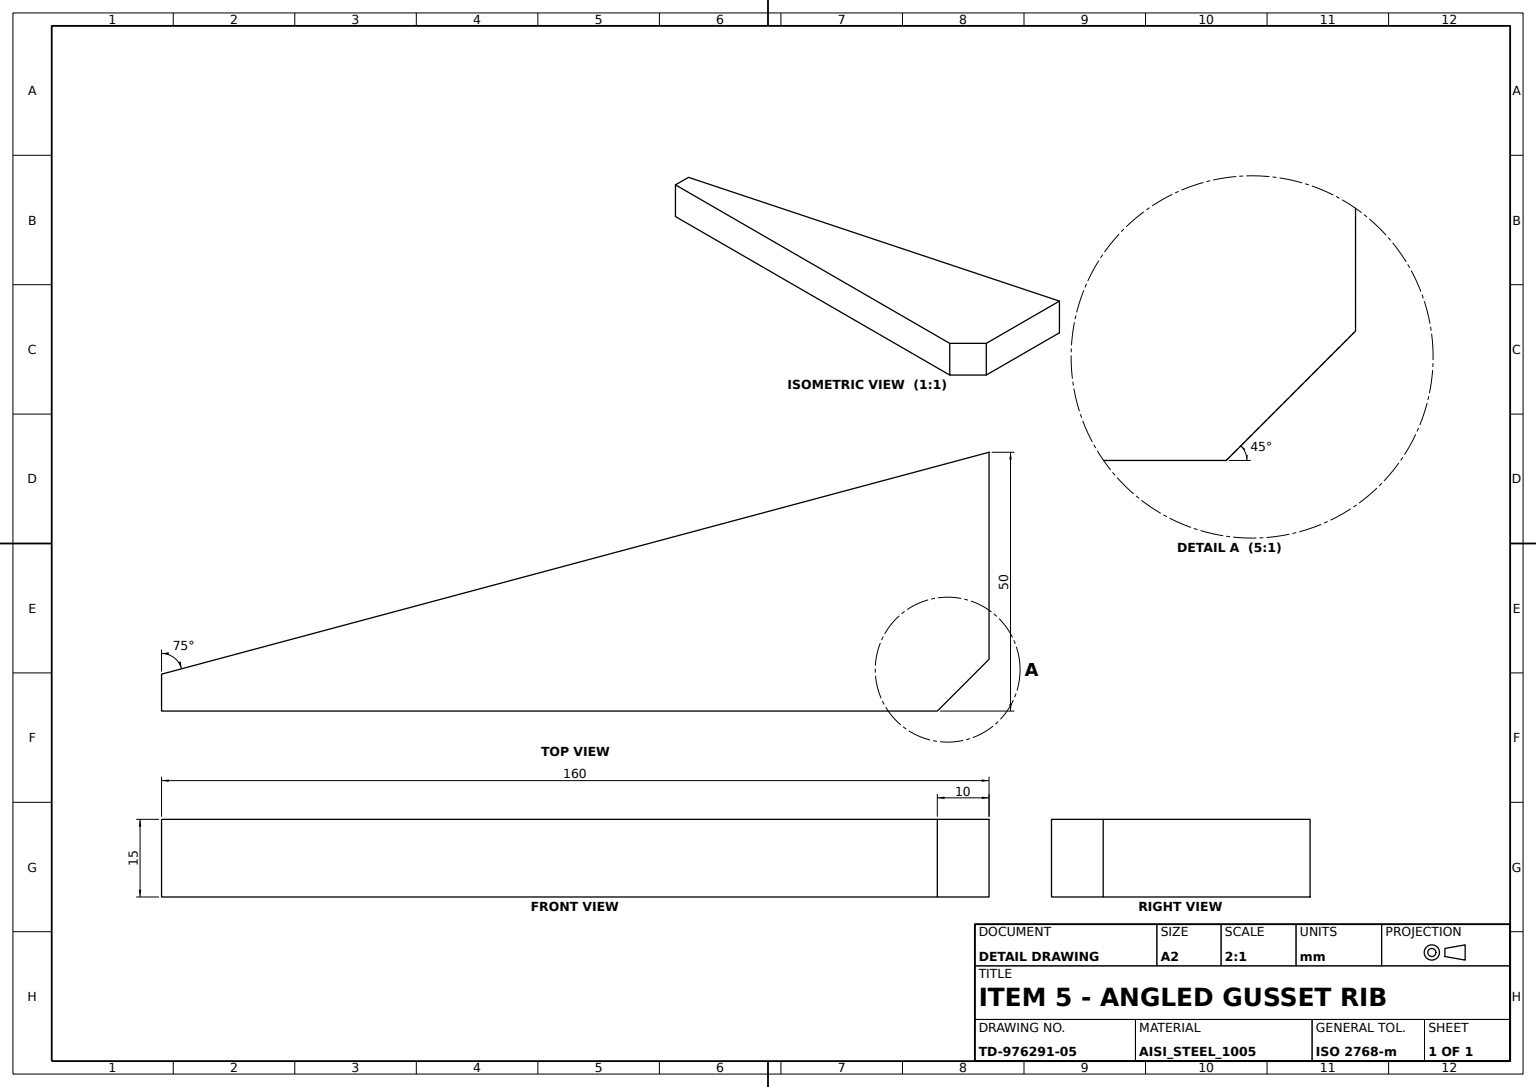
ISO-10303-21;
HEADER;
FILE_DESCRIPTION((''),'2;1');
FILE_NAME('','',(''),(''),'','','');
FILE_SCHEMA(('AUTOMOTIVE_DESIGN'));
ENDSEC;
DATA;
#1=APPLICATION_CONTEXT('');
#2=PRODUCT_CONTEXT('',#1,'mechanical');
#3=PRODUCT('','','',(#2));
#4=PRODUCT_DEFINITION_FORMATION('','',#3);
#5=PRODUCT_DEFINITION_CONTEXT('',#1,'design');
#6=PRODUCT_DEFINITION('','',#4,#5);
#7=PRODUCT_DEFINITION_SHAPE('','',#6);
#8=(LENGTH_UNIT()NAMED_UNIT(*)SI_UNIT(.MILLI.,.METRE.));
#9=(NAMED_UNIT(*)PLANE_ANGLE_UNIT()SI_UNIT($,.RADIAN.));
#10=(NAMED_UNIT(*)SI_UNIT($,.STERADIAN.)SOLID_ANGLE_UNIT());
#11=UNCERTAINTY_MEASURE_WITH_UNIT(LENGTH_MEASURE(0.005),#8,'distance_accuracy_value','');
#12=(GEOMETRIC_REPRESENTATION_CONTEXT(3)GLOBAL_UNCERTAINTY_ASSIGNED_CONTEXT((#11))GLOBAL_UNIT_ASSIGNED_CONTEXT((#8,#9,#10))REPRESENTATION_CONTEXT('',''));
#13=CARTESIAN_POINT('',(0.,-7.128129,160.));
#14=VERTEX_POINT('',#13);
#15=CARTESIAN_POINT('',(0.,-50.,0.));
#16=VERTEX_POINT('',#15);
#17=DIRECTION('',(0.,-0.258819045,-0.965925826));
#18=VECTOR('',#17,1000.);
#19=LINE('',#13,#18);
#20=EDGE_CURVE('',#14,#16,#19,.T.);
#21=ORIENTED_EDGE('',*,*,#20,.T.);
#22=CARTESIAN_POINT('',(0.,-10.,0.));
#23=VERTEX_POINT('',#22);
#24=DIRECTION('',(0.,1.,0.));
#25=VECTOR('',#24,1000.);
#26=LINE('',#15,#25);
#27=EDGE_CURVE('',#16,#23,#26,.T.);
#28=ORIENTED_EDGE('',*,*,#27,.T.);
#29=CARTESIAN_POINT('',(0.,0.,10.));
#30=VERTEX_POINT('',#29);
#31=DIRECTION('',(0.,0.707106781,0.707106781));
#32=VECTOR('',#31,1000.);
#33=LINE('',#22,#32);
#34=EDGE_CURVE('',#23,#30,#33,.T.);
#35=ORIENTED_EDGE('',*,*,#34,.T.);
#36=CARTESIAN_POINT('',(0.,0.,160.));
#37=VERTEX_POINT('',#36);
#38=DIRECTION('',(0.,0.,1.));
#39=VECTOR('',#38,1000.);
#40=LINE('',#29,#39);
#41=EDGE_CURVE('',#30,#37,#40,.T.);
#42=ORIENTED_EDGE('',*,*,#41,.T.);
#43=DIRECTION('',(0.,-1.,0.));
#44=VECTOR('',#43,1000.);
#45=LINE('',#36,#44);
#46=EDGE_CURVE('',#37,#14,#45,.T.);
#47=ORIENTED_EDGE('',*,*,#46,.T.);
#48=EDGE_LOOP('',(#21,#28,#35,#42,#47));
#49=FACE_BOUND('',#48,.T.);
#50=CARTESIAN_POINT('',(0.,0.,0.));
#51=DIRECTION('',(1.,0.,0.));
#52=DIRECTION('',(0.,0.,-1.));
#53=AXIS2_PLACEMENT_3D('',#50,#51,#52);
#54=PLANE('',#53);
#55=ADVANCED_FACE('',(#49),#54,.T.);
#56=CARTESIAN_POINT('',(-15.,0.,160.));
#57=VERTEX_POINT('',#56);
#58=VECTOR('',#51,1000.);
#59=LINE('',#56,#58);
#60=EDGE_CURVE('',#57,#37,#59,.T.);
#61=ORIENTED_EDGE('',*,*,#60,.T.);
#62=ORIENTED_EDGE('',*,*,#41,.F.);
#63=CARTESIAN_POINT('',(-15.,0.,10.));
#64=VERTEX_POINT('',#63);
#65=LINE('',#63,#58);
#66=EDGE_CURVE('',#64,#30,#65,.T.);
#67=ORIENTED_EDGE('',*,*,#66,.F.);
#68=LINE('',#63,#39);
#69=EDGE_CURVE('',#64,#57,#68,.T.);
#70=ORIENTED_EDGE('',*,*,#69,.T.);
#71=EDGE_LOOP('',(#61,#62,#67,#70));
#72=FACE_BOUND('',#71,.T.);
#73=AXIS2_PLACEMENT_3D('',#63,#24,#38);
#74=PLANE('',#73);
#75=ADVANCED_FACE('',(#72),#74,.T.);
#76=CARTESIAN_POINT('',(-15.,-7.128129,160.));
#77=VERTEX_POINT('',#76);
#78=LINE('',#56,#44);
#79=EDGE_CURVE('',#57,#77,#78,.T.);
#80=ORIENTED_EDGE('',*,*,#79,.T.);
#81=LINE('',#76,#58);
#82=EDGE_CURVE('',#77,#14,#81,.T.);
#83=ORIENTED_EDGE('',*,*,#82,.T.);
#84=ORIENTED_EDGE('',*,*,#46,.F.);
#85=ORIENTED_EDGE('',*,*,#60,.F.);
#86=EDGE_LOOP('',(#80,#83,#84,#85));
#87=FACE_BOUND('',#86,.T.);
#88=AXIS2_PLACEMENT_3D('',#56,#38,#51);
#89=PLANE('',#88);
#90=ADVANCED_FACE('',(#87),#89,.T.);
#91=CARTESIAN_POINT('',(-15.,-10.,0.));
#92=VERTEX_POINT('',#91);
#93=LINE('',#91,#32);
#94=EDGE_CURVE('',#92,#64,#93,.T.);
#95=ORIENTED_EDGE('',*,*,#94,.T.);
#96=ORIENTED_EDGE('',*,*,#66,.T.);
#97=ORIENTED_EDGE('',*,*,#34,.F.);
#98=LINE('',#91,#58);
#99=EDGE_CURVE('',#92,#23,#98,.T.);
#100=ORIENTED_EDGE('',*,*,#99,.F.);
#101=EDGE_LOOP('',(#95,#96,#97,#100));
#102=FACE_BOUND('',#101,.T.);
#103=DIRECTION('',(0.,0.707106781,-0.707106781));
#104=AXIS2_PLACEMENT_3D('',#91,#103,#31);
#105=PLANE('',#104);
#106=ADVANCED_FACE('',(#102),#105,.T.);
#107=ORIENTED_EDGE('',*,*,#94,.F.);
#108=CARTESIAN_POINT('',(-15.,-50.,0.));
#109=VERTEX_POINT('',#108);
#110=LINE('',#108,#25);
#111=EDGE_CURVE('',#109,#92,#110,.T.);
#112=ORIENTED_EDGE('',*,*,#111,.F.);
#113=LINE('',#76,#18);
#114=EDGE_CURVE('',#77,#109,#113,.T.);
#115=ORIENTED_EDGE('',*,*,#114,.F.);
#116=ORIENTED_EDGE('',*,*,#79,.F.);
#117=ORIENTED_EDGE('',*,*,#69,.F.);
#118=EDGE_LOOP('',(#107,#112,#115,#116,#117));
#119=FACE_BOUND('',#118,.T.);
#120=CARTESIAN_POINT('',(-15.,0.,0.));
#121=AXIS2_PLACEMENT_3D('',#120,#51,#52);
#122=PLANE('',#121);
#123=ADVANCED_FACE('',(#119),#122,.F.);
#124=ORIENTED_EDGE('',*,*,#20,.F.);
#125=ORIENTED_EDGE('',*,*,#82,.F.);
#126=ORIENTED_EDGE('',*,*,#114,.T.);
#127=LINE('',#108,#58);
#128=EDGE_CURVE('',#109,#16,#127,.T.);
#129=ORIENTED_EDGE('',*,*,#128,.T.);
#130=EDGE_LOOP('',(#124,#125,#126,#129));
#131=FACE_BOUND('',#130,.T.);
#132=DIRECTION('',(0.,-0.965925826,0.258819045));
#133=AXIS2_PLACEMENT_3D('',#76,#132,#17);
#134=PLANE('',#133);
#135=ADVANCED_FACE('',(#131),#134,.T.);
#136=ORIENTED_EDGE('',*,*,#27,.F.);
#137=ORIENTED_EDGE('',*,*,#128,.F.);
#138=ORIENTED_EDGE('',*,*,#111,.T.);
#139=ORIENTED_EDGE('',*,*,#99,.T.);
#140=EDGE_LOOP('',(#136,#137,#138,#139));
#141=FACE_BOUND('',#140,.T.);
#142=DIRECTION('',(-1.,0.,0.));
#143=AXIS2_PLACEMENT_3D('',#108,#52,#142);
#144=PLANE('',#143);
#145=ADVANCED_FACE('',(#141),#144,.T.);
#146=CLOSED_SHELL('',(#55,#75,#90,#106,#123,#135,#145));
#147=MANIFOLD_SOLID_BREP('',#146);
#148=ADVANCED_BREP_SHAPE_REPRESENTATION('',(#147),#12);
#149=SHAPE_DEFINITION_REPRESENTATION(#7,#148);
ENDSEC;
END-ISO-10303-21;
